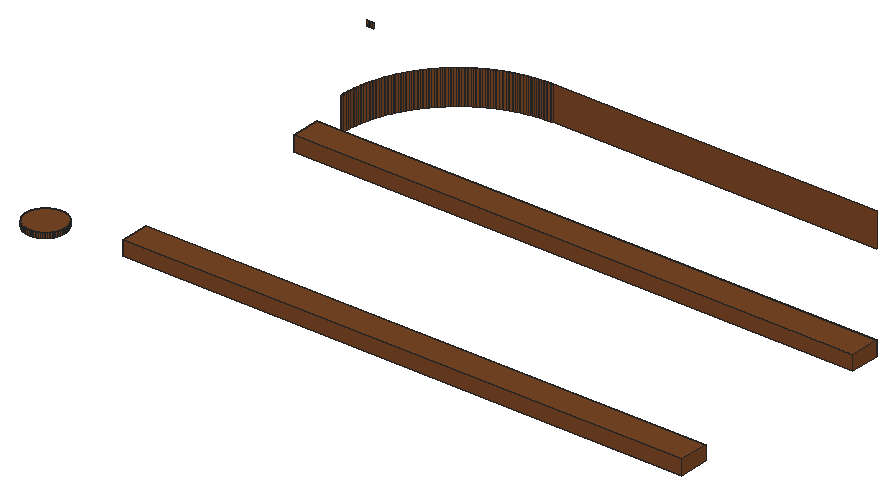
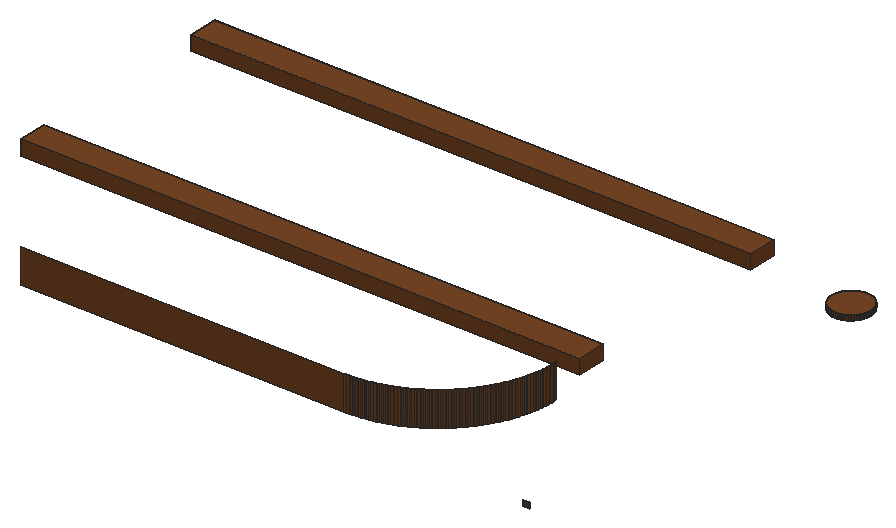
# SketchUp Ruby script. Lengths in inches.
U = 1.inch
M = Sketchup.active_model
def pt(a) = Geom::Point3d.new(a.map { |v| v * U })
def face(e, loops, mat)
  f = e.add_face(loops[0].map { |a| pt(a) })
  loops[1..].each { |l| e.add_face(l.map { |a| pt(a) }).erase! }
  f.material = f.back_material = mat if mat
  f
end
# faces: each face lists its corners as indices into pts; further lists are holes
def faces(e, pts, list, mat = nil) = list.each { |f| face(e, (f[0].is_a?(Array) ? f : [f]).map { |l| l.map { |i| pts[i] } }, mat) }
# xy, xz, yz: faces in a plane at the given z, y or x. An outline is a flat list of corners, or four numbers for a rectangle; further outlines are holes
def ring(l) = l.size == 4 ? [[l[0], l[1]], [l[2], l[1]], [l[2], l[3]], [l[0], l[3]]] : l.each_slice(2).to_a
def flat(e, list, mat, &to3) = list.each { |f| face(e, (f[0].is_a?(Array) ? f : [f]).map { |l| ring(l).map { |u, v| to3.(u, v) } }, mat) }
def xy(e, z, list, mat = nil) = flat(e, list, mat) { |x, y| [x, y, z] }
def xz(e, y, list, mat = nil) = flat(e, list, mat) { |x, z| [x, y, z] }
def yz(e, x, list, mat = nil) = flat(e, list, mat) { |y, z| [x, y, z] }
def lines(e, pts, list) = list.each { |a, b| e.add_line(pt(pts[a]), pt(pts[b])) }
# prism: a flat outline (further loops are holes) pulled along v
def prism(e, loops, v, mat = nil)
  f = face(e, loops, mat); d = Geom::Vector3d.new(v.map { |x| x * U })
  f.pushpull(f.normal.samedirection?(d) ? d.length : -d.length)
end
def box(e, o, s, mat = nil) = prism(e, [[o, [o[0] + s[0], o[1], o[2]], [o[0] + s[0], o[1] + s[1], o[2]], [o[0], o[1] + s[1], o[2]]]], [0, 0, s[2]], mat)
def at(x, y, z, deg = 0) = Geom::Transformation.translation(pt([x, y, z])) * Geom::Transformation.rotation(ORIGIN, Z_AXIS, deg.degrees)
def axes(o, x, y, z) = Geom::Transformation.new([*x, 0, *y, 0, *z, 0, *pt(o).to_a, 1])
def part(name) = M.definitions.add(name)
# library, detail: a bought-in or finely detailed component or shape, given as its bounding box
def library(name, o, s) = part(name).tap { |d| box(d.entities, o, s) }
def detail(e, o, s) = box(e.add_group.entities, o, s)
def put(e, d, t, mat = nil) = e.add_instance(d, t).tap { |i| i.material = mat if mat }
def group(e, t, mat = nil) = e.add_group.tap { |g| g.transformation = t; g.material = mat if mat }.entities
root = M.entities
M.materials.add("[Wood Veneer 01]3").color = [120, 70, 37]
c1 = part("8")
box(c1.entities,[0,0,0],[3,1.5,57],"[Wood Veneer 01]3")
xy(root,118.5,[[71.82,124.67,71.74,124.68,71.65,124.7,71.57,124.71,71.49,124.73,71.41,124.76,71.33,124.78,71.25,124.8125,71.17,124.85,71.1,124.88,71.02,124.92,70.95,124.96,70.88,125.01,70.8125,125.06,70.75,125.11,70.68,125.16,70.62,125.22,70.5625,125.28,70.5,125.34,70.45,125.4,70.3,125.61,70.22,125.75,70.18,125.83,70.15,125.9,70.12,125.98,70.09,126.0625,70.07,126.14,70.05,126.22,70.03,126.31,70.01,126.47,70,126.56,70,126.81,70.02,126.97,70.04,127.06,70.1,127.3,70.16,127.45,70.2,127.53,70.23,127.61,70.27,127.68,70.42,127.89,70.47,127.95,70.52,128.02,70.58,128.08,70.64,128.13,70.7,128.19,70.84,128.29,70.9,128.34,70.98,128.38,71.05,128.43,71.125,128.46,71.2,128.5,71.44,128.59,71.52,128.61,71.68,128.64,71.76,128.65,71.85,128.66,71.93,128.67,72.01,128.67,72.1,128.66,72.18,128.66,72.26,128.65,72.35,128.64,72.59,128.58,72.83,128.49,72.9,128.45,72.98,128.41,73.05,128.37,73.12,128.32,73.1875,128.28,73.25,128.23,73.32,128.17,73.38,128.11,73.4375,128.06,73.5,127.99,73.55,127.93,73.6,127.86,73.65,127.8,73.7,127.73,73.74,127.65,73.82,127.51,73.91,127.27,73.97,127.03,73.98,126.94,74,126.78,74,126.53,73.99,126.44,73.98,126.36,73.9,126.04,73.84,125.88,73.8,125.8,73.77,125.73,73.73,125.65,73.63,125.51,73.58,125.45,73.53,125.38,73.48,125.32,73.3,125.14,73.16,125.04,73.1,124.99,73.02,124.95,72.95,124.91,72.8,124.83,72.64,124.77,72.32,124.69,72.24,124.68,72.15,124.67]],"[Wood Veneer 01]3")
xz(root,124.67,[[71.82,118,71.9,118.5],[71.9,118,71.99,118.5],[71.99,118,72.07,118.5],[72.07,118,72.15,118.5]],"[Wood Veneer 01]3")
xz(root,128.66,[[72.1,118,72.18,118.5]],"[Wood Veneer 01]3")
xz(root,128.67,[[71.93,118,72.01,118.5]],"[Wood Veneer 01]3")
xz(root,165,[[92.6875,118,92.84,121.5],[92.84,118,93,121.5],[93,118,126,121.5]],"[Wood Veneer 01]3")
xz(root,168,[[71.9,118,71.99,118.5],[71.99,118,72.07,118.5]],"[Wood Veneer 01]3")
xz(root,168.01,[[72.15,118,72.24,118.5]],"[Wood Veneer 01]3")
yz(root,70,[[126.56,118,126.64,118.5],[126.64,118,126.72,118.5],[126.72,118,126.81,118.5]],"[Wood Veneer 01]3")
yz(root,74,[[126.53,118,126.61,118.5],[126.61,118,126.69,118.5],[126.69,118,126.78,118.5]],"[Wood Veneer 01]3")
yz(root,81,[[153,118,153.16,121.5],[153.16,118,153.3125,121.5]],"[Wood Veneer 01]3")
p = [[71.49,124.73,118],[71.41,124.76,118],[71.41,124.76,118.5],[71.49,124.73,118.5],[71.57,124.71,118],[71.57,124.71,118.5],
  [71.65,124.7,118],[71.65,124.7,118.5],[71.82,124.67,118],[71.74,124.68,118],[71.74,124.68,118.5],[71.82,124.67,118.5],
  [72.24,124.68,118],[72.15,124.67,118],[72.15,124.67,118.5],[72.24,124.68,118.5],[72.32,124.69,118],[72.32,124.69,118.5],
  [72.4,124.71,118],[72.4,124.71,118.5],[72.48,124.73,118],[72.48,124.73,118.5],[72.56,124.75,118],[72.56,124.75,118.5],
  [72.64,124.77,118],[72.64,124.77,118.5],[71.17,124.85,118],[71.1,124.88,118],[71.1,124.88,118.5],[71.17,124.85,118.5],
  [71.25,124.8125,118],[71.25,124.8125,118.5],[71.33,124.78,118],[71.33,124.78,118.5],[72.72,124.8,118],[72.72,124.8,118.5],
  [72.8,124.83,118],[72.8,124.83,118.5],[72.875,124.87,118],[72.875,124.87,118.5],[71.02,124.92,118],[71.02,124.92,118.5],
  [70.95,124.96,118],[70.95,124.96,118.5],[72.95,124.91,118],[72.95,124.91,118.5],[73.02,124.95,118],[73.02,124.95,118.5],
  [73.1,124.99,118],[73.1,124.99,118.5],[70.88,125.01,118],[70.8125,125.06,118],[70.8125,125.06,118.5],[70.88,125.01,118.5],
  [73.16,125.04,118],[73.16,125.04,118.5],[73.23,125.09,118],[73.23,125.09,118.5],[70.75,125.11,118],[70.75,125.11,118.5],
  [70.68,125.16,118],[70.68,125.16,118.5],[73.3,125.14,118],[73.3,125.14,118.5],[73.36,125.2,118],[73.36,125.2,118.5],
  [70.62,125.22,118],[70.62,125.22,118.5],[70.5625,125.28,118],[70.5625,125.28,118.5],[73.42,125.26,118],[73.42,125.26,118.5],
  [70.5,125.34,118],[70.5,125.34,118.5],[70.45,125.4,118],[70.45,125.4,118.5],[73.48,125.32,118],[73.48,125.32,118.5],
  [73.53,125.38,118],[73.53,125.38,118.5],[70.4,125.47,118],[70.4,125.47,118.5],[73.58,125.45,118],[73.58,125.45,118.5],
  [73.63,125.51,118],[73.63,125.51,118.5],[70.35,125.54,118],[70.35,125.54,118.5],[70.3,125.61,118],[70.3,125.61,118.5],
  [73.68,125.58,118],[73.68,125.58,118.5],[70.26,125.68,118],[70.26,125.68,118.5],[73.73,125.65,118],[73.73,125.65,118.5],
  [70.22,125.75,118],[70.22,125.75,118.5],[73.77,125.73,118],[73.77,125.73,118.5],[73.8,125.8,118],[73.8,125.8,118.5],
  [70.18,125.83,118],[70.18,125.83,118.5],[70.15,125.9,118],[70.15,125.9,118.5],[73.84,125.88,118],[73.84,125.88,118.5],
  [70.12,125.98,118],[70.12,125.98,118.5],[73.87,125.96,118],[73.87,125.96,118.5],[70.09,126.0625,118],[70.09,126.0625,118.5],
  [73.9,126.04,118],[73.9,126.04,118.5],[73.92,126.12,118],[73.92,126.12,118.5],[70.07,126.14,118],[70.05,126.22,118],
  [70.05,126.22,118.5],[70.07,126.14,118.5],[73.94,126.2,118],[73.94,126.2,118.5],[70.03,126.31,118],[70.03,126.31,118.5],
  [73.96,126.28,118],[73.96,126.28,118.5],[70.02,126.39,118],[70.02,126.39,118.5],[73.98,126.36,118],[73.98,126.36,118.5],
  [70.01,126.47,118],[70.01,126.47,118.5],[73.99,126.44,118],[73.99,126.44,118.5],[74,126.53,118],[74,126.53,118.5],
  [70,126.56,118],[70,126.56,118.5],[70,126.81,118],[70.01,126.89,118],[70.01,126.89,118.5],[70,126.81,118.5],
  [73.99,126.86,118],[74,126.78,118],[74,126.78,118.5],[73.99,126.86,118.5],[70.02,126.97,118],[70.02,126.97,118.5],
  [73.98,126.94,118],[73.98,126.94,118.5],[73.97,127.03,118],[73.97,127.03,118.5],[70.04,127.06,118],[70.04,127.06,118.5],
  [73.95,127.11,118],[73.95,127.11,118.5],[70.06,127.14,118],[70.06,127.14,118.5],[70.08,127.22,118],[70.08,127.22,118.5],
  [73.93,127.19,118],[73.93,127.19,118.5],[70.1,127.3,118],[70.1,127.3,118.5],[73.91,127.27,118],[73.91,127.27,118.5],
  [70.13,127.375,118],[70.13,127.375,118.5],[73.88,127.35,118],[73.88,127.35,118.5],[70.16,127.45,118],[70.16,127.45,118.5],
  [73.85,127.43,118],[73.85,127.43,118.5],[73.82,127.51,118],[73.82,127.51,118.5],[70.2,127.53,118],[70.2,127.53,118.5],
  [70.23,127.61,118],[70.23,127.61,118.5],[73.78,127.58,118],[73.78,127.58,118.5],[70.27,127.68,118],[70.27,127.68,118.5],
  [73.74,127.65,118],[73.74,127.65,118.5],[70.32,127.75,118],[70.32,127.75,118.5],[73.7,127.73,118],[73.7,127.73,118.5],
  [73.65,127.8,118],[73.65,127.8,118.5],[70.37,127.82,118],[70.37,127.82,118.5],[70.42,127.89,118],[70.42,127.89,118.5],
  [73.6,127.86,118],[73.6,127.86,118.5],[70.47,127.95,118],[70.47,127.95,118.5],[73.55,127.93,118],[73.55,127.93,118.5],
  [73.5,127.99,118],[73.5,127.99,118.5],[70.52,128.02,118],[70.52,128.02,118.5],[70.58,128.08,118],[70.58,128.08,118.5],
  [73.4375,128.06,118],[73.4375,128.06,118.5],[70.64,128.13,118],[70.64,128.13,118.5],[70.7,128.19,118],[70.7,128.19,118.5],
  [73.32,128.17,118],[73.38,128.11,118],[73.38,128.11,118.5],[73.32,128.17,118.5],[70.77,128.24,118],[70.77,128.24,118.5],
  [70.84,128.29,118],[70.84,128.29,118.5],[73.1875,128.28,118],[73.25,128.23,118],[73.25,128.23,118.5],[73.1875,128.28,118.5],
  [70.9,128.34,118],[70.9,128.34,118.5],[70.98,128.38,118],[70.98,128.38,118.5],[73.05,128.37,118],[73.12,128.32,118],
  [73.12,128.32,118.5],[73.05,128.37,118.5],[71.05,128.43,118],[71.05,128.43,118.5],[71.125,128.46,118],[71.125,128.46,118.5],
  [72.9,128.45,118],[72.98,128.41,118],[72.98,128.41,118.5],[72.9,128.45,118.5],[71.2,128.5,118],[71.2,128.5,118.5],
  [71.28,128.53,118],[71.28,128.53,118.5],[71.36,128.56,118],[71.36,128.56,118.5],[72.75,128.52,118],[72.83,128.49,118],
  [72.83,128.49,118.5],[72.75,128.52,118.5],[72.67,128.55,118],[72.67,128.55,118.5],[71.44,128.59,118],[71.44,128.59,118.5],
  [71.52,128.61,118],[71.52,128.61,118.5],[71.6,128.625,118],[71.6,128.625,118.5],[71.68,128.64,118],[71.68,128.64,118.5],
  [71.76,128.65,118],[71.76,128.65,118.5],[72.18,128.66,118],[72.26,128.65,118],[72.26,128.65,118.5],[72.18,128.66,118.5],
  [72.35,128.64,118],[72.43,128.62,118],[72.43,128.62,118.5],[72.35,128.64,118.5],[72.51,128.6,118],[72.51,128.6,118.5],
  [72.59,128.58,118],[72.59,128.58,118.5],[71.85,128.66,118],[71.85,128.66,118.5],[71.93,128.67,118],[71.93,128.67,118.5],
  [72.01,128.67,118],[72.1,128.66,118],[72.1,128.66,118.5],[72.01,128.67,118.5],[81.01,153.47,118],[81.01,153.47,121],
  [81.01,153.47,121.5],[81,153.3125,121.5],[81,153.3125,121],[81,153.3125,118],[81.02,153.63,118],[81.02,153.63,121],
  [81.02,153.63,121.5],[81.03,153.78,118],[81.03,153.78,121],[81.03,153.78,121.5],[81.04,153.94,118],[81.04,153.94,121],
  [81.04,153.94,121.5],[81.05,154.1,118],[81.05,154.1,121],[81.05,154.1,121.5],[81.07,154.25,118],[81.07,154.25,121],
  [81.07,154.25,121.5],[81.08,154.41,118],[81.08,154.41,121],[81.08,154.41,121.5],[81.1,154.57,118],[81.1,154.57,121],
  [81.1,154.57,121.5],[81.125,154.72,118],[81.125,154.72,121],[81.125,154.72,121.5],[81.15,154.88,118],[81.15,154.88,121],
  [81.15,154.88,121.5],[81.17,155.03,118],[81.17,155.03,121],[81.17,155.03,121.5],[81.2,155.1875,118],[81.2,155.1875,121],
  [81.2,155.1875,121.5],[81.23,155.34,118],[81.23,155.34,121],[81.23,155.34,121.5],[81.26,155.49,118],[81.26,155.49,121],
  [81.26,155.49,121.5],[81.3,155.65,118],[81.3,155.65,121],[81.3,155.65,121.5],[81.33,155.8,118],[81.33,155.8,121],
  [81.33,155.8,121.5],[81.37,155.95,118],[81.37,155.95,121],[81.37,155.95,121.5],[81.41,156.11,118],[81.41,156.11,121],
  [81.41,156.11,121.5],[81.45,156.26,118],[81.45,156.26,121],[81.45,156.26,121.5],[81.49,156.41,118],[81.49,156.41,121],
  [81.49,156.41,121.5],[81.54,156.56,118],[81.54,156.56,121],[81.54,156.56,121.5],[81.59,156.71,118],[81.59,156.71,121],
  [81.59,156.71,121.5],[81.64,156.86,118],[81.64,156.86,121],[81.64,156.86,121.5],[81.6875,157.01,118],[81.6875,157.01,121],
  [81.6875,157.01,121.5],[81.74,157.15,118],[81.74,157.15,121],[81.74,157.15,121.5],[81.8,157.3,118],[81.8,157.3,121],
  [81.8,157.3,121.5],[81.85,157.45,118],[81.85,157.45,121],[81.85,157.45,121.5],[81.91,157.59,118],[81.91,157.59,121],
  [81.91,157.59,121.5],[81.97,157.74,118],[81.97,157.74,121],[81.97,157.74,121.5],[82.04,157.88,118],[82.04,157.88,121],
  [82.04,157.88,121.5],[82.1,158.02,118],[82.1,158.02,121],[82.1,158.02,121.5],[82.17,158.17,118],[82.17,158.17,121],
  [82.17,158.17,121.5],[82.24,158.31,118],[82.24,158.31,121],[82.24,158.31,121.5],[82.31,158.45,118],[82.31,158.45,121],
  [82.31,158.45,121.5],[82.38,158.59,118],[82.38,158.59,121],[82.38,158.59,121.5],[82.45,158.73,118],[82.45,158.73,121],
  [82.45,158.73,121.5],[82.53,158.86,118],[82.53,158.86,121],[82.53,158.86,121.5],[82.61,159,118],[82.61,159,121],
  [82.61,159,121.5],[82.6875,159.14,118],[82.6875,159.14,121],[82.6875,159.14,121.5],[82.77,159.27,118],[82.77,159.27,121],
  [82.77,159.27,121.5],[82.85,159.4,118],[82.85,159.4,121],[82.85,159.4,121.5],[82.9375,159.54,118],[82.9375,159.54,121],
  [82.9375,159.54,121.5],[83.02,159.67,118],[83.02,159.67,121],[83.02,159.67,121.5],[83.11,159.8,118],[83.11,159.8,121],
  [83.11,159.8,121.5],[83.2,159.93,118],[83.2,159.93,121],[83.2,159.93,121.5],[83.29,160.05,118],[83.29,160.05,121],
  [83.29,160.05,121.5],[83.38,160.18,118],[83.38,160.18,121],[83.38,160.18,121.5],[83.48,160.31,118],[83.48,160.31,121],
  [83.48,160.31,121.5],[83.58,160.43,118],[83.58,160.43,121],[83.58,160.43,121.5],[83.67,160.55,118],[83.67,160.55,121],
  [83.67,160.55,121.5],[83.77,160.67,118],[83.77,160.67,121],[83.77,160.67,121.5],[83.875,160.79,118],[83.875,160.79,121],
  [83.875,160.79,121.5],[83.98,160.91,118],[83.98,160.91,121],[83.98,160.91,121.5],[84.08,161.03,118],[84.08,161.03,121],
  [84.08,161.03,121.5],[84.1875,161.15,118],[84.1875,161.15,121],[84.1875,161.15,121.5],[84.3,161.26,118],[84.3,161.26,121],
  [84.3,161.26,121.5],[84.4,161.375,118],[84.4,161.375,121],[84.4,161.375,121.5],[84.51,161.49,118],[84.51,161.49,121],
  [84.51,161.49,121.5],[84.625,161.6,118],[84.625,161.6,121],[84.625,161.6,121.5],[84.74,161.7,118],[84.74,161.7,121],
  [84.74,161.7,121.5],[84.85,161.8125,118],[84.85,161.8125,121],[84.85,161.8125,121.5],[84.97,161.92,118],[84.97,161.92,121],
  [84.97,161.92,121.5],[85.09,162.02,118],[85.09,162.02,121],[85.09,162.02,121.5],[85.21,162.125,118],[85.21,162.125,121],
  [85.21,162.125,121.5],[85.33,162.23,118],[85.33,162.23,121],[85.33,162.23,121.5],[85.45,162.33,118],[85.45,162.33,121],
  [85.45,162.33,121.5],[85.57,162.42,118],[85.57,162.42,121],[85.57,162.42,121.5],[85.69,162.52,118],[85.69,162.52,121],
  [85.69,162.52,121.5],[85.82,162.62,118],[85.82,162.62,121],[85.82,162.62,121.5],[85.95,162.71,118],[85.95,162.71,121],
  [85.95,162.71,121.5],[86.07,162.8,118],[86.07,162.8,121],[86.07,162.8,121.5],[86.2,162.89,118],[86.2,162.89,121],
  [86.2,162.89,121.5],[86.33,162.98,118],[86.33,162.98,121],[86.33,162.98,121.5],[86.46,163.0625,118],[86.46,163.0625,121],
  [86.46,163.0625,121.5],[86.6,163.15,118],[86.6,163.15,121],[86.6,163.15,121.5],[86.73,163.23,118],[86.73,163.23,121],
  [86.73,163.23,121.5],[86.86,163.3125,118],[86.86,163.3125,121],[86.86,163.3125,121.5],[87,163.39,118],[87,163.39,121],
  [87,163.39,121.5],[87.14,163.47,118],[87.14,163.47,121],[87.14,163.47,121.5],[87.27,163.55,118],[87.27,163.55,121],
  [87.27,163.55,121.5],[87.41,163.62,118],[87.41,163.62,121],[87.41,163.62,121.5],[87.55,163.69,118],[87.55,163.69,121],
  [87.55,163.69,121.5],[87.69,163.76,118],[87.69,163.76,121],[87.69,163.76,121.5],[87.83,163.83,118],[87.83,163.83,121],
  [87.83,163.83,121.5],[87.98,163.9,118],[87.98,163.9,121],[87.98,163.9,121.5],[88.12,163.96,118],[88.12,163.96,121],
  [88.12,163.96,121.5],[88.26,164.03,118],[88.26,164.03,121],[88.26,164.03,121.5],[88.41,164.09,118],[88.41,164.09,121],
  [88.41,164.09,121.5],[88.55,164.15,118],[88.55,164.15,121],[88.55,164.15,121.5],[88.7,164.2,118],[88.7,164.2,121],
  [88.7,164.2,121.5],[88.85,164.26,118],[88.85,164.26,121],[88.85,164.26,121.5],[88.99,164.3125,118],[88.99,164.3125,121],
  [88.99,164.3125,121.5],[89.14,164.36,118],[89.14,164.36,121],[89.14,164.36,121.5],[89.29,164.41,118],[89.29,164.41,121],
  [89.29,164.41,121.5],[89.44,164.46,118],[89.44,164.46,121],[89.44,164.46,121.5],[89.59,164.51,118],[89.59,164.51,121],
  [89.59,164.51,121.5],[89.74,164.55,118],[89.74,164.55,121],[89.74,164.55,121.5],[89.89,164.59,118],[89.89,164.59,121],
  [89.89,164.59,121.5],[90.05,164.63,118],[90.05,164.63,121],[90.05,164.63,121.5],[90.2,164.67,118],[90.2,164.67,121],
  [90.2,164.67,121.5],[90.35,164.7,118],[90.35,164.7,121],[90.35,164.7,121.5],[90.51,164.74,118],[90.51,164.74,121],
  [90.51,164.74,121.5],[90.66,164.77,118],[90.66,164.77,121],[90.66,164.77,121.5],[90.8125,164.8,118],[90.8125,164.8,121],
  [90.8125,164.8,121.5],[90.97,164.83,118],[90.97,164.83,121],[90.97,164.83,121.5],[91.12,164.85,118],[91.12,164.85,121],
  [91.12,164.85,121.5],[91.28,164.875,118],[91.28,164.875,121],[91.28,164.875,121.5],[91.43,164.9,118],[91.43,164.9,121],
  [91.43,164.9,121.5],[91.59,164.92,118],[91.59,164.92,121],[91.59,164.92,121.5],[91.75,164.93,118],[91.75,164.93,121],
  [91.75,164.93,121.5],[91.9,164.95,118],[91.9,164.95,121],[91.9,164.95,121.5],[92.06,164.96,118],[92.06,164.96,121],
  [92.06,164.96,121.5],[92.22,164.97,118],[92.22,164.97,121],[92.22,164.97,121.5],[92.37,164.98,118],[92.37,164.98,121],
  [92.37,164.98,121.5],[92.53,164.99,118],[92.53,164.99,121],[92.53,164.99,121.5],[92.6875,165,118],[92.6875,165,121],
  [92.6875,165,121.5],[71.82,168.01,118],[71.74,168.02,118],[71.74,168.02,118.5],[71.82,168.01,118.5],[71.65,168.03,118],
  [71.65,168.03,118.5],[71.9,168,118],[71.9,168,118.5],[72.15,168.01,118],[72.07,168,118],[72.07,168,118.5],
  [72.15,168.01,118.5],[72.32,168.03,118],[72.24,168.01,118],[72.24,168.01,118.5],[72.32,168.03,118.5],[72.4,168.04,118],
  [72.4,168.04,118.5]]
faces(root,p,[[0,1,2,3],[4,0,3,5],[6,4,5,7],[8,9,10,11],[9,6,7,10],[12,13,14,15],[16,12,15,17],[18,16,17,19],
  [20,18,19,21],[22,20,21,23],[24,22,23,25],[26,27,28,29],[30,26,29,31],[1,32,33,2],[32,30,31,33],[34,24,25,35],
  [36,34,35,37],[38,36,37,39],[27,40,41,28],[40,42,43,41],[44,38,39,45],[46,44,45,47],[48,46,47,49],[50,51,52,53],
  [42,50,53,43],[54,48,49,55],[56,54,55,57],[51,58,59,52],[58,60,61,59],[62,56,57,63],[64,62,63,65],[60,66,67,61],
  [66,68,69,67],[70,64,65,71],[68,72,73,69],[72,74,75,73],[76,70,71,77],[78,76,77,79],[74,80,81,75],[82,78,79,83],
  [84,82,83,85],[80,86,87,81],[86,88,89,87],[90,84,85,91],[88,92,93,89],[94,90,91,95],[92,96,97,93],[98,94,95,99],
  [100,98,99,101],[96,102,103,97],[102,104,105,103],[106,100,101,107],[104,108,109,105],[110,106,107,111],[108,112,113,109],[114,110,111,115],
  [116,114,115,117],[118,119,120,121],[112,118,121,113],[122,116,117,123],[119,124,125,120],[126,122,123,127],[124,128,129,125],[130,126,127,131],
  [128,132,133,129],[134,130,131,135],[136,134,135,137],[132,138,139,133],[140,141,142,143],[144,145,146,147],[141,148,149,142],[150,144,147,151],
  [152,150,151,153],[148,154,155,149],[156,152,153,157],[154,158,159,155],[158,160,161,159],[162,156,157,163],[160,164,165,161],[166,162,163,167],
  [164,168,169,165],[170,166,167,171],[168,172,173,169],[174,170,171,175],[176,174,175,177],[172,178,179,173],[178,180,181,179],[182,176,177,183],
  [180,184,185,181],[186,182,183,187],[184,188,189,185],[190,186,187,191],[192,190,191,193],[188,194,195,189],[194,196,197,195],[198,192,193,199],
  [196,200,201,197],[202,198,199,203],[204,202,203,205],[200,206,207,201],[206,208,209,207],[210,204,205,211],[208,212,213,209],[212,214,215,213],
  [216,217,218,219],[217,210,211,218],[214,220,221,215],[220,222,223,221],[224,225,226,227],[225,216,219,226],[222,228,229,223],[228,230,231,229],
  [232,233,234,235],[233,224,227,234],[230,236,237,231],[236,238,239,237],[240,241,242,243],[241,232,235,242],[238,244,245,239],[244,246,247,245],
  [246,248,249,247],[250,251,252,253],[254,250,253,255],[251,240,243,252],[248,256,257,249],[256,258,259,257],[258,260,261,259],[260,262,263,261],
  [262,264,265,263],[266,267,268,269],[270,271,272,273],[267,270,273,268],[271,274,275,272],[274,276,277,275],[276,254,255,277],[264,278,279,265],
  [278,280,281,279],[282,283,284,285],[286,287,288,289,290,291],[292,293,294,288,287,286],[295,296,297,294,293,292],[298,299,300,297,296,295],[301,302,303,300,299,298],[304,305,306,303,302,301],
  [307,308,309,306,305,304],[310,311,312,309,308,307],[313,314,315,312,311,310],[316,317,318,315,314,313],[319,320,321,318,317,316],[322,323,324,321,320,319],[325,326,327,324,323,322],[328,329,330,327,326,325],
  [331,332,333,330,329,328],[334,335,336,333,332,331],[337,338,339,336,335,334],[340,341,342,339,338,337],[343,344,345,342,341,340],[346,347,348,345,344,343],[349,350,351,348,347,346],[352,353,354,351,350,349],
  [355,356,357,354,353,352],[358,359,360,357,356,355],[361,362,363,360,359,358],[364,365,366,363,362,361],[367,368,369,366,365,364],[370,371,372,369,368,367],[373,374,375,372,371,370],[376,377,378,375,374,373],
  [379,380,381,378,377,376],[382,383,384,381,380,379],[385,386,387,384,383,382],[388,389,390,387,386,385],[391,392,393,390,389,388],[394,395,396,393,392,391],[397,398,399,396,395,394],[400,401,402,399,398,397],
  [403,404,405,402,401,400],[406,407,408,405,404,403],[409,410,411,408,407,406],[412,413,414,411,410,409],[415,416,417,414,413,412],[418,419,420,417,416,415],[421,422,423,420,419,418],[424,425,426,423,422,421],
  [427,428,429,426,425,424],[430,431,432,429,428,427],[433,434,435,432,431,430],[436,437,438,435,434,433],[439,440,441,438,437,436],[442,443,444,441,440,439],[445,446,447,444,443,442],[448,449,450,447,446,445],
  [451,452,453,450,449,448],[454,455,456,453,452,451],[457,458,459,456,455,454],[460,461,462,459,458,457],[463,464,465,462,461,460],[466,467,468,465,464,463],[469,470,471,468,467,466],[472,473,474,471,470,469],
  [475,476,477,474,473,472],[478,479,480,477,476,475],[481,482,483,480,479,478],[484,485,486,483,482,481],[487,488,489,486,485,484],[490,491,492,489,488,487],[493,494,495,492,491,490],[496,497,498,495,494,493],
  [499,500,501,498,497,496],[502,503,504,501,500,499],[505,506,507,504,503,502],[508,509,510,507,506,505],[511,512,513,510,509,508],[514,515,516,513,512,511],[517,518,519,516,515,514],[520,521,522,519,518,517],
  [523,524,525,522,521,520],[526,527,528,525,524,523],[529,530,531,528,527,526],[532,533,534,531,530,529],[535,536,537,534,533,532],[538,539,540,537,536,535],[541,542,543,540,539,538],[544,545,546,543,542,541],
  [547,548,549,546,545,544],[550,551,552,549,548,547],[553,554,555,552,551,550],[556,557,558,555,554,553],[559,560,561,558,557,556],[562,563,564,561,560,559],[565,566,567,564,563,562],[568,569,570,567,566,565],
  [571,572,573,570,569,568],[574,575,576,573,572,571],[577,578,579,576,575,574],[580,581,582,579,578,577],[583,584,585,582,581,580],[586,587,588,585,584,583],[589,590,591,588,587,586],[592,593,594,591,590,589],
  [595,596,597,594,593,592],[598,599,600,597,596,595],[601,602,603,600,599,598],[604,605,606,603,602,601],[607,608,609,606,605,604],[610,611,612,609,608,607],[613,614,615,612,611,610],[616,617,618,615,614,613],
  [619,620,621,618,617,616],[622,623,624,621,620,619],[625,626,627,624,623,622],[628,629,630,627,626,625],[631,632,633,630,629,628],[634,635,636,633,632,631],[637,638,639,640],[638,641,642,639],
  [643,637,640,644],[645,646,647,648],[649,650,651,652],[653,649,652,654]],"[Wood Veneer 01]3")
put(root,c1,axes([81,125.25,119],[0,1,0],[0,0,1],[1,0,0]))
put(root,c1,axes([81,147,119],[0,1,0],[0,0,1],[1,0,0]))
